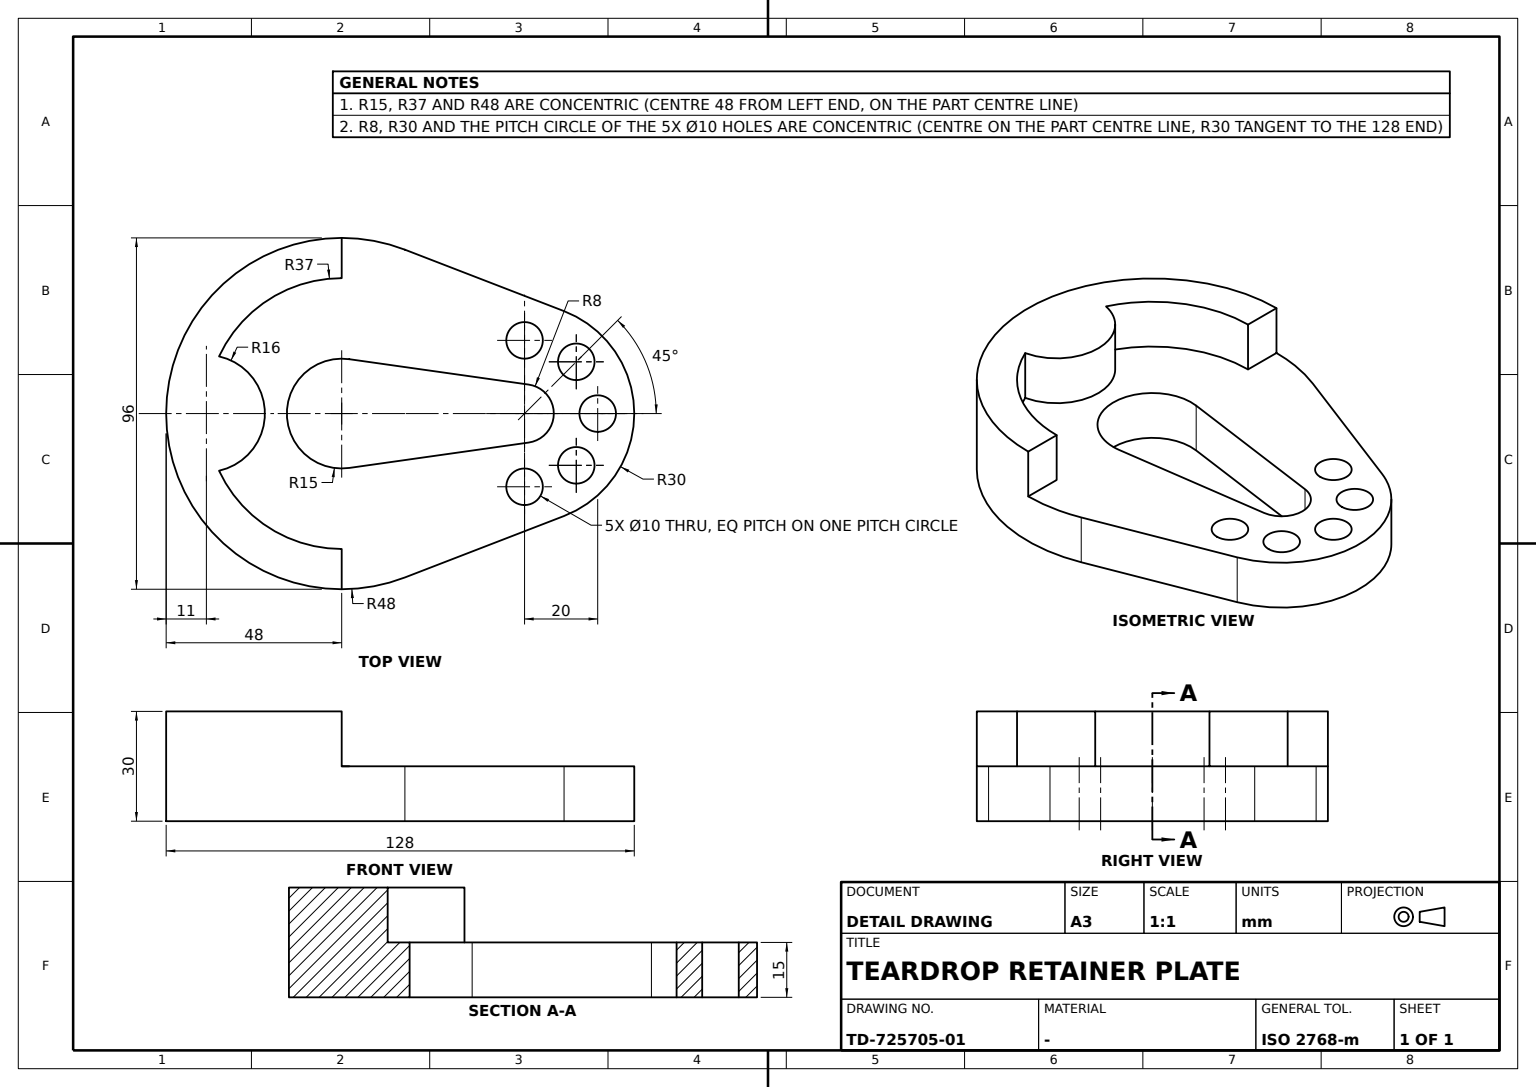
ISO-10303-21;
HEADER;
FILE_DESCRIPTION((''),'2;1');
FILE_NAME('','',(''),(''),'','','');
FILE_SCHEMA(('AUTOMOTIVE_DESIGN'));
ENDSEC;
DATA;
#1=APPLICATION_CONTEXT('');
#2=PRODUCT_CONTEXT('',#1,'mechanical');
#3=PRODUCT('','','',(#2));
#4=PRODUCT_DEFINITION_FORMATION('','',#3);
#5=PRODUCT_DEFINITION_CONTEXT('',#1,'design');
#6=PRODUCT_DEFINITION('','',#4,#5);
#7=PRODUCT_DEFINITION_SHAPE('','',#6);
#8=(LENGTH_UNIT()NAMED_UNIT(*)SI_UNIT(.MILLI.,.METRE.));
#9=(NAMED_UNIT(*)PLANE_ANGLE_UNIT()SI_UNIT($,.RADIAN.));
#10=(NAMED_UNIT(*)SI_UNIT($,.STERADIAN.)SOLID_ANGLE_UNIT());
#11=UNCERTAINTY_MEASURE_WITH_UNIT(LENGTH_MEASURE(0.005),#8,'distance_accuracy_value','');
#12=(GEOMETRIC_REPRESENTATION_CONTEXT(3)GLOBAL_UNCERTAINTY_ASSIGNED_CONTEXT((#11))GLOBAL_UNIT_ASSIGNED_CONTEXT((#8,#9,#10))REPRESENTATION_CONTEXT('',''));
#13=CARTESIAN_POINT('',(7.921212,51.12,0.));
#14=VERTEX_POINT('',#13);
#15=CARTESIAN_POINT('',(-7.921212,51.12,0.));
#16=VERTEX_POINT('',#15);
#17=CARTESIAN_POINT('',(0.,50.,0.));
#18=DIRECTION('',(0.,0.,1.));
#19=DIRECTION('',(1.,0.,0.));
#20=AXIS2_PLACEMENT_3D('',#17,#18,#19);
#21=CIRCLE('',#20,8.);
#22=EDGE_CURVE('',#14,#16,#21,.T.);
#23=ORIENTED_EDGE('',*,*,#22,.T.);
#24=CARTESIAN_POINT('',(-7.921212,51.12,-15.));
#25=VERTEX_POINT('',#24);
#26=CARTESIAN_POINT('',(-7.921212,51.12,-7.5));
#27=VECTOR('',#18,1000.);
#28=LINE('',#26,#27);
#29=EDGE_CURVE('',#16,#25,#28,.F.);
#30=ORIENTED_EDGE('',*,*,#29,.T.);
#31=CARTESIAN_POINT('',(7.921212,51.12,-15.));
#32=VERTEX_POINT('',#31);
#33=CARTESIAN_POINT('',(0.,50.,-15.));
#34=AXIS2_PLACEMENT_3D('',#33,#18,#19);
#35=CIRCLE('',#34,8.);
#36=EDGE_CURVE('',#32,#25,#35,.T.);
#37=ORIENTED_EDGE('',*,*,#36,.F.);
#38=CARTESIAN_POINT('',(7.921212,51.12,-7.5));
#39=LINE('',#38,#27);
#40=EDGE_CURVE('',#14,#32,#39,.F.);
#41=ORIENTED_EDGE('',*,*,#40,.F.);
#42=EDGE_LOOP('',(#23,#30,#37,#41));
#43=FACE_BOUND('',#42,.T.);
#44=CARTESIAN_POINT('',(0.,50.,-7.5));
#45=AXIS2_PLACEMENT_3D('',#44,#18,#19);
#46=CYLINDRICAL_SURFACE('',#45,8.);
#47=ADVANCED_FACE('',(#43),#46,.F.);
#48=CARTESIAN_POINT('',(19.142136,64.142136,-15.));
#49=VERTEX_POINT('',#48);
#50=CARTESIAN_POINT('',(14.142136,64.142136,-15.));
#51=AXIS2_PLACEMENT_3D('',#50,#18,#19);
#52=CIRCLE('',#51,5.);
#53=EDGE_CURVE('',#49,#49,#52,.T.);
#54=ORIENTED_EDGE('',*,*,#53,.T.);
#55=EDGE_LOOP('',(#54));
#56=FACE_BOUND('',#55,.T.);
#57=CARTESIAN_POINT('',(-44.781711,17.28,-15.));
#58=VERTEX_POINT('',#57);
#59=CARTESIAN_POINT('',(44.781711,17.28,-15.));
#60=VERTEX_POINT('',#59);
#61=CARTESIAN_POINT('',(0.,0.,-15.));
#62=AXIS2_PLACEMENT_3D('',#61,#18,#19);
#63=CIRCLE('',#62,48.);
#64=EDGE_CURVE('',#58,#60,#63,.T.);
#65=ORIENTED_EDGE('',*,*,#64,.F.);
#66=CARTESIAN_POINT('',(-27.988569,60.8,-15.));
#67=VERTEX_POINT('',#66);
#68=DIRECTION('',(0.36,0.932952303,0.));
#69=VECTOR('',#68,1000.);
#70=LINE('',#57,#69);
#71=EDGE_CURVE('',#58,#67,#70,.T.);
#72=ORIENTED_EDGE('',*,*,#71,.T.);
#73=CARTESIAN_POINT('',(27.988569,60.8,-15.));
#74=VERTEX_POINT('',#73);
#75=CIRCLE('',#34,30.);
#76=EDGE_CURVE('',#74,#67,#75,.T.);
#77=ORIENTED_EDGE('',*,*,#76,.F.);
#78=DIRECTION('',(0.36,-0.932952303,0.));
#79=VECTOR('',#78,1000.);
#80=LINE('',#73,#79);
#81=EDGE_CURVE('',#74,#60,#80,.T.);
#82=ORIENTED_EDGE('',*,*,#81,.T.);
#83=EDGE_LOOP('',(#65,#72,#77,#82));
#84=FACE_BOUND('',#83,.T.);
#85=CARTESIAN_POINT('',(-15.,50.,-15.));
#86=VERTEX_POINT('',#85);
#87=CARTESIAN_POINT('',(-20.,50.,-15.));
#88=AXIS2_PLACEMENT_3D('',#87,#18,#19);
#89=CIRCLE('',#88,5.);
#90=EDGE_CURVE('',#86,#86,#89,.T.);
#91=ORIENTED_EDGE('',*,*,#90,.T.);
#92=EDGE_LOOP('',(#91));
#93=FACE_BOUND('',#92,.T.);
#94=CARTESIAN_POINT('',(5.,70.,-15.));
#95=VERTEX_POINT('',#94);
#96=CARTESIAN_POINT('',(0.,70.,-15.));
#97=AXIS2_PLACEMENT_3D('',#96,#18,#19);
#98=CIRCLE('',#97,5.);
#99=EDGE_CURVE('',#95,#95,#98,.T.);
#100=ORIENTED_EDGE('',*,*,#99,.T.);
#101=EDGE_LOOP('',(#100));
#102=FACE_BOUND('',#101,.T.);
#103=CARTESIAN_POINT('',(25.,50.,-15.));
#104=VERTEX_POINT('',#103);
#105=CARTESIAN_POINT('',(20.,50.,-15.));
#106=AXIS2_PLACEMENT_3D('',#105,#18,#19);
#107=CIRCLE('',#106,5.);
#108=EDGE_CURVE('',#104,#104,#107,.T.);
#109=ORIENTED_EDGE('',*,*,#108,.T.);
#110=EDGE_LOOP('',(#109));
#111=FACE_BOUND('',#110,.T.);
#112=CARTESIAN_POINT('',(-9.142136,64.142136,-15.));
#113=VERTEX_POINT('',#112);
#114=CARTESIAN_POINT('',(-14.142136,64.142136,-15.));
#115=AXIS2_PLACEMENT_3D('',#114,#18,#19);
#116=CIRCLE('',#115,5.);
#117=EDGE_CURVE('',#113,#113,#116,.T.);
#118=ORIENTED_EDGE('',*,*,#117,.T.);
#119=EDGE_LOOP('',(#118));
#120=FACE_BOUND('',#119,.T.);
#121=CARTESIAN_POINT('',(-14.852273,2.1,-15.));
#122=VERTEX_POINT('',#121);
#123=CARTESIAN_POINT('',(14.852273,2.1,-15.));
#124=VERTEX_POINT('',#123);
#125=CIRCLE('',#62,15.);
#126=EDGE_CURVE('',#122,#124,#125,.T.);
#127=ORIENTED_EDGE('',*,*,#126,.T.);
#128=DIRECTION('',(0.14,-0.990151504,0.));
#129=VECTOR('',#128,1000.);
#130=LINE('',#31,#129);
#131=EDGE_CURVE('',#32,#124,#130,.T.);
#132=ORIENTED_EDGE('',*,*,#131,.F.);
#133=ORIENTED_EDGE('',*,*,#36,.T.);
#134=DIRECTION('',(0.14,0.990151504,0.));
#135=VECTOR('',#134,1000.);
#136=LINE('',#121,#135);
#137=EDGE_CURVE('',#122,#25,#136,.T.);
#138=ORIENTED_EDGE('',*,*,#137,.F.);
#139=EDGE_LOOP('',(#127,#132,#133,#138));
#140=FACE_BOUND('',#139,.T.);
#141=PLANE('',#62);
#142=ADVANCED_FACE('',(#56,#84,#93,#102,#111,#120,#140),#141,.F.);
#143=CARTESIAN_POINT('',(25.,50.,0.));
#144=VERTEX_POINT('',#143);
#145=CARTESIAN_POINT('',(20.,50.,0.));
#146=AXIS2_PLACEMENT_3D('',#145,#18,#19);
#147=CIRCLE('',#146,5.);
#148=EDGE_CURVE('',#144,#144,#147,.T.);
#149=ORIENTED_EDGE('',*,*,#148,.T.);
#150=EDGE_LOOP('',(#149));
#151=FACE_BOUND('',#150,.T.);
#152=ORIENTED_EDGE('',*,*,#108,.F.);
#153=EDGE_LOOP('',(#152));
#154=FACE_BOUND('',#153,.T.);
#155=CARTESIAN_POINT('',(20.,50.,-7.5));
#156=AXIS2_PLACEMENT_3D('',#155,#18,#19);
#157=CYLINDRICAL_SURFACE('',#156,5.);
#158=ADVANCED_FACE('',(#151,#154),#157,.F.);
#159=CARTESIAN_POINT('',(27.988569,60.8,0.));
#160=VERTEX_POINT('',#159);
#161=CARTESIAN_POINT('',(44.781711,17.28,0.));
#162=VERTEX_POINT('',#161);
#163=LINE('',#159,#79);
#164=EDGE_CURVE('',#160,#162,#163,.T.);
#165=ORIENTED_EDGE('',*,*,#164,.T.);
#166=CARTESIAN_POINT('',(44.781711,17.28,-7.5));
#167=LINE('',#166,#27);
#168=EDGE_CURVE('',#162,#60,#167,.F.);
#169=ORIENTED_EDGE('',*,*,#168,.T.);
#170=ORIENTED_EDGE('',*,*,#81,.F.);
#171=CARTESIAN_POINT('',(27.988569,60.8,-7.5));
#172=LINE('',#171,#27);
#173=EDGE_CURVE('',#160,#74,#172,.F.);
#174=ORIENTED_EDGE('',*,*,#173,.F.);
#175=EDGE_LOOP('',(#165,#169,#170,#174));
#176=FACE_BOUND('',#175,.T.);
#177=DIRECTION('',(0.932952303,0.36,0.));
#178=AXIS2_PLACEMENT_3D('',#159,#177,#78);
#179=PLANE('',#178);
#180=ADVANCED_FACE('',(#176),#179,.T.);
#181=ORIENTED_EDGE('',*,*,#71,.F.);
#182=CARTESIAN_POINT('',(-44.781711,17.28,0.));
#183=VERTEX_POINT('',#182);
#184=CARTESIAN_POINT('',(-44.781711,17.28,-7.5));
#185=LINE('',#184,#27);
#186=EDGE_CURVE('',#183,#58,#185,.F.);
#187=ORIENTED_EDGE('',*,*,#186,.F.);
#188=CARTESIAN_POINT('',(-27.988569,60.8,0.));
#189=VERTEX_POINT('',#188);
#190=LINE('',#182,#69);
#191=EDGE_CURVE('',#183,#189,#190,.T.);
#192=ORIENTED_EDGE('',*,*,#191,.T.);
#193=CARTESIAN_POINT('',(-27.988569,60.8,-7.5));
#194=LINE('',#193,#27);
#195=EDGE_CURVE('',#189,#67,#194,.F.);
#196=ORIENTED_EDGE('',*,*,#195,.T.);
#197=EDGE_LOOP('',(#181,#187,#192,#196));
#198=FACE_BOUND('',#197,.T.);
#199=DIRECTION('',(-0.932952303,0.36,0.));
#200=AXIS2_PLACEMENT_3D('',#182,#199,#68);
#201=PLANE('',#200);
#202=ADVANCED_FACE('',(#198),#201,.T.);
#203=CARTESIAN_POINT('',(15.621528,-33.540541,15.));
#204=VERTEX_POINT('',#203);
#205=CARTESIAN_POINT('',(-15.621528,-33.540541,15.));
#206=VERTEX_POINT('',#205);
#207=CARTESIAN_POINT('',(0.,-37.,15.));
#208=AXIS2_PLACEMENT_3D('',#207,#18,#19);
#209=CIRCLE('',#208,16.);
#210=EDGE_CURVE('',#204,#206,#209,.T.);
#211=ORIENTED_EDGE('',*,*,#210,.F.);
#212=CARTESIAN_POINT('',(15.621528,-33.540541,0.));
#213=VERTEX_POINT('',#212);
#214=LINE('',#212,#27);
#215=EDGE_CURVE('',#213,#204,#214,.T.);
#216=ORIENTED_EDGE('',*,*,#215,.F.);
#217=CARTESIAN_POINT('',(-15.621528,-33.540541,0.));
#218=VERTEX_POINT('',#217);
#219=CARTESIAN_POINT('',(0.,-37.,0.));
#220=AXIS2_PLACEMENT_3D('',#219,#18,#19);
#221=CIRCLE('',#220,16.);
#222=EDGE_CURVE('',#213,#218,#221,.T.);
#223=ORIENTED_EDGE('',*,*,#222,.T.);
#224=LINE('',#217,#27);
#225=EDGE_CURVE('',#218,#206,#224,.T.);
#226=ORIENTED_EDGE('',*,*,#225,.T.);
#227=EDGE_LOOP('',(#211,#216,#223,#226));
#228=FACE_BOUND('',#227,.T.);
#229=CARTESIAN_POINT('',(0.,-37.,7.5));
#230=AXIS2_PLACEMENT_3D('',#229,#18,#19);
#231=CYLINDRICAL_SURFACE('',#230,16.);
#232=ADVANCED_FACE('',(#228),#231,.T.);
#233=CARTESIAN_POINT('',(48.,0.,0.));
#234=VERTEX_POINT('',#233);
#235=CARTESIAN_POINT('',(48.,0.,15.));
#236=VERTEX_POINT('',#235);
#237=LINE('',#233,#27);
#238=EDGE_CURVE('',#234,#236,#237,.T.);
#239=ORIENTED_EDGE('',*,*,#238,.F.);
#240=CARTESIAN_POINT('',(37.,0.,0.));
#241=VERTEX_POINT('',#240);
#242=CARTESIAN_POINT('',(0.,0.,0.));
#243=DIRECTION('',(-1.,0.,0.));
#244=VECTOR('',#243,1000.);
#245=LINE('',#242,#244);
#246=EDGE_CURVE('',#234,#241,#245,.T.);
#247=ORIENTED_EDGE('',*,*,#246,.T.);
#248=CARTESIAN_POINT('',(37.,0.,15.));
#249=VERTEX_POINT('',#248);
#250=LINE('',#240,#27);
#251=EDGE_CURVE('',#241,#249,#250,.T.);
#252=ORIENTED_EDGE('',*,*,#251,.T.);
#253=CARTESIAN_POINT('',(0.,0.,15.));
#254=LINE('',#253,#244);
#255=EDGE_CURVE('',#236,#249,#254,.T.);
#256=ORIENTED_EDGE('',*,*,#255,.F.);
#257=EDGE_LOOP('',(#239,#247,#252,#256));
#258=FACE_BOUND('',#257,.T.);
#259=DIRECTION('',(0.,1.,0.));
#260=AXIS2_PLACEMENT_3D('',#233,#259,#243);
#261=PLANE('',#260);
#262=ADVANCED_FACE('',(#258),#261,.T.);
#263=CARTESIAN_POINT('',(-15.,50.,0.));
#264=VERTEX_POINT('',#263);
#265=CARTESIAN_POINT('',(-20.,50.,0.));
#266=AXIS2_PLACEMENT_3D('',#265,#18,#19);
#267=CIRCLE('',#266,5.);
#268=EDGE_CURVE('',#264,#264,#267,.T.);
#269=ORIENTED_EDGE('',*,*,#268,.T.);
#270=EDGE_LOOP('',(#269));
#271=FACE_BOUND('',#270,.T.);
#272=ORIENTED_EDGE('',*,*,#90,.F.);
#273=EDGE_LOOP('',(#272));
#274=FACE_BOUND('',#273,.T.);
#275=CARTESIAN_POINT('',(-20.,50.,-7.5));
#276=AXIS2_PLACEMENT_3D('',#275,#18,#19);
#277=CYLINDRICAL_SURFACE('',#276,5.);
#278=ADVANCED_FACE('',(#271,#274),#277,.F.);
#279=ORIENTED_EDGE('',*,*,#29,.F.);
#280=CARTESIAN_POINT('',(-14.852273,2.1,0.));
#281=VERTEX_POINT('',#280);
#282=LINE('',#280,#135);
#283=EDGE_CURVE('',#281,#16,#282,.T.);
#284=ORIENTED_EDGE('',*,*,#283,.F.);
#285=CARTESIAN_POINT('',(-14.852273,2.1,-7.5));
#286=LINE('',#285,#27);
#287=EDGE_CURVE('',#281,#122,#286,.F.);
#288=ORIENTED_EDGE('',*,*,#287,.T.);
#289=ORIENTED_EDGE('',*,*,#137,.T.);
#290=EDGE_LOOP('',(#279,#284,#288,#289));
#291=FACE_BOUND('',#290,.T.);
#292=DIRECTION('',(-0.990151504,0.14,0.));
#293=AXIS2_PLACEMENT_3D('',#280,#292,#134);
#294=PLANE('',#293);
#295=ADVANCED_FACE('',(#291),#294,.F.);
#296=ORIENTED_EDGE('',*,*,#131,.T.);
#297=CARTESIAN_POINT('',(14.852273,2.1,0.));
#298=VERTEX_POINT('',#297);
#299=CARTESIAN_POINT('',(14.852273,2.1,-7.5));
#300=LINE('',#299,#27);
#301=EDGE_CURVE('',#298,#124,#300,.F.);
#302=ORIENTED_EDGE('',*,*,#301,.F.);
#303=LINE('',#13,#129);
#304=EDGE_CURVE('',#14,#298,#303,.T.);
#305=ORIENTED_EDGE('',*,*,#304,.F.);
#306=ORIENTED_EDGE('',*,*,#40,.T.);
#307=EDGE_LOOP('',(#296,#302,#305,#306));
#308=FACE_BOUND('',#307,.T.);
#309=DIRECTION('',(0.990151504,0.14,0.));
#310=AXIS2_PLACEMENT_3D('',#13,#309,#128);
#311=PLANE('',#310);
#312=ADVANCED_FACE('',(#308),#311,.F.);
#313=ORIENTED_EDGE('',*,*,#99,.F.);
#314=EDGE_LOOP('',(#313));
#315=FACE_BOUND('',#314,.T.);
#316=CARTESIAN_POINT('',(5.,70.,0.));
#317=VERTEX_POINT('',#316);
#318=CARTESIAN_POINT('',(0.,70.,0.));
#319=AXIS2_PLACEMENT_3D('',#318,#18,#19);
#320=CIRCLE('',#319,5.);
#321=EDGE_CURVE('',#317,#317,#320,.T.);
#322=ORIENTED_EDGE('',*,*,#321,.T.);
#323=EDGE_LOOP('',(#322));
#324=FACE_BOUND('',#323,.T.);
#325=CARTESIAN_POINT('',(0.,70.,-7.5));
#326=AXIS2_PLACEMENT_3D('',#325,#18,#19);
#327=CYLINDRICAL_SURFACE('',#326,5.);
#328=ADVANCED_FACE('',(#315,#324),#327,.F.);
#329=CARTESIAN_POINT('',(-37.,0.,0.));
#330=VERTEX_POINT('',#329);
#331=CARTESIAN_POINT('',(-48.,0.,0.));
#332=VERTEX_POINT('',#331);
#333=EDGE_CURVE('',#330,#332,#245,.T.);
#334=ORIENTED_EDGE('',*,*,#333,.T.);
#335=CARTESIAN_POINT('',(-48.,0.,15.));
#336=VERTEX_POINT('',#335);
#337=LINE('',#331,#27);
#338=EDGE_CURVE('',#332,#336,#337,.T.);
#339=ORIENTED_EDGE('',*,*,#338,.T.);
#340=CARTESIAN_POINT('',(-37.,0.,15.));
#341=VERTEX_POINT('',#340);
#342=EDGE_CURVE('',#341,#336,#254,.T.);
#343=ORIENTED_EDGE('',*,*,#342,.F.);
#344=LINE('',#329,#27);
#345=EDGE_CURVE('',#330,#341,#344,.T.);
#346=ORIENTED_EDGE('',*,*,#345,.F.);
#347=EDGE_LOOP('',(#334,#339,#343,#346));
#348=FACE_BOUND('',#347,.T.);
#349=ADVANCED_FACE('',(#348),#261,.T.);
#350=AXIS2_PLACEMENT_3D('',#242,#18,#19);
#351=CIRCLE('',#350,15.);
#352=EDGE_CURVE('',#281,#298,#351,.T.);
#353=ORIENTED_EDGE('',*,*,#352,.T.);
#354=ORIENTED_EDGE('',*,*,#301,.T.);
#355=ORIENTED_EDGE('',*,*,#126,.F.);
#356=ORIENTED_EDGE('',*,*,#287,.F.);
#357=EDGE_LOOP('',(#353,#354,#355,#356));
#358=FACE_BOUND('',#357,.T.);
#359=CARTESIAN_POINT('',(0.,0.,-7.5));
#360=AXIS2_PLACEMENT_3D('',#359,#18,#19);
#361=CYLINDRICAL_SURFACE('',#360,15.);
#362=ADVANCED_FACE('',(#358),#361,.F.);
#363=ORIENTED_EDGE('',*,*,#246,.F.);
#364=CIRCLE('',#350,48.);
#365=EDGE_CURVE('',#234,#162,#364,.T.);
#366=ORIENTED_EDGE('',*,*,#365,.T.);
#367=ORIENTED_EDGE('',*,*,#164,.F.);
#368=CIRCLE('',#20,30.);
#369=EDGE_CURVE('',#160,#189,#368,.T.);
#370=ORIENTED_EDGE('',*,*,#369,.T.);
#371=ORIENTED_EDGE('',*,*,#191,.F.);
#372=EDGE_CURVE('',#183,#332,#364,.T.);
#373=ORIENTED_EDGE('',*,*,#372,.T.);
#374=ORIENTED_EDGE('',*,*,#333,.F.);
#375=CIRCLE('',#350,37.);
#376=EDGE_CURVE('',#330,#218,#375,.T.);
#377=ORIENTED_EDGE('',*,*,#376,.T.);
#378=ORIENTED_EDGE('',*,*,#222,.F.);
#379=EDGE_CURVE('',#213,#241,#375,.T.);
#380=ORIENTED_EDGE('',*,*,#379,.T.);
#381=EDGE_LOOP('',(#363,#366,#367,#370,#371,#373,#374,#377,#378,#380));
#382=FACE_BOUND('',#381,.T.);
#383=ORIENTED_EDGE('',*,*,#283,.T.);
#384=ORIENTED_EDGE('',*,*,#22,.F.);
#385=ORIENTED_EDGE('',*,*,#304,.T.);
#386=ORIENTED_EDGE('',*,*,#352,.F.);
#387=EDGE_LOOP('',(#383,#384,#385,#386));
#388=FACE_BOUND('',#387,.T.);
#389=CARTESIAN_POINT('',(-9.142136,64.142136,0.));
#390=VERTEX_POINT('',#389);
#391=CARTESIAN_POINT('',(-14.142136,64.142136,0.));
#392=AXIS2_PLACEMENT_3D('',#391,#18,#19);
#393=CIRCLE('',#392,5.);
#394=EDGE_CURVE('',#390,#390,#393,.T.);
#395=ORIENTED_EDGE('',*,*,#394,.F.);
#396=EDGE_LOOP('',(#395));
#397=FACE_BOUND('',#396,.T.);
#398=ORIENTED_EDGE('',*,*,#148,.F.);
#399=EDGE_LOOP('',(#398));
#400=FACE_BOUND('',#399,.T.);
#401=ORIENTED_EDGE('',*,*,#268,.F.);
#402=EDGE_LOOP('',(#401));
#403=FACE_BOUND('',#402,.T.);
#404=CARTESIAN_POINT('',(19.142136,64.142136,0.));
#405=VERTEX_POINT('',#404);
#406=CARTESIAN_POINT('',(14.142136,64.142136,0.));
#407=AXIS2_PLACEMENT_3D('',#406,#18,#19);
#408=CIRCLE('',#407,5.);
#409=EDGE_CURVE('',#405,#405,#408,.T.);
#410=ORIENTED_EDGE('',*,*,#409,.F.);
#411=EDGE_LOOP('',(#410));
#412=FACE_BOUND('',#411,.T.);
#413=ORIENTED_EDGE('',*,*,#321,.F.);
#414=EDGE_LOOP('',(#413));
#415=FACE_BOUND('',#414,.T.);
#416=PLANE('',#350);
#417=ADVANCED_FACE('',(#382,#388,#397,#400,#403,#412,#415),#416,.T.);
#418=ORIENTED_EDGE('',*,*,#409,.T.);
#419=EDGE_LOOP('',(#418));
#420=FACE_BOUND('',#419,.T.);
#421=ORIENTED_EDGE('',*,*,#53,.F.);
#422=EDGE_LOOP('',(#421));
#423=FACE_BOUND('',#422,.T.);
#424=CARTESIAN_POINT('',(14.142136,64.142136,-7.5));
#425=AXIS2_PLACEMENT_3D('',#424,#18,#19);
#426=CYLINDRICAL_SURFACE('',#425,5.);
#427=ADVANCED_FACE('',(#420,#423),#426,.F.);
#428=ORIENTED_EDGE('',*,*,#251,.F.);
#429=ORIENTED_EDGE('',*,*,#379,.F.);
#430=ORIENTED_EDGE('',*,*,#215,.T.);
#431=AXIS2_PLACEMENT_3D('',#253,#18,#19);
#432=CIRCLE('',#431,37.);
#433=EDGE_CURVE('',#204,#249,#432,.T.);
#434=ORIENTED_EDGE('',*,*,#433,.T.);
#435=EDGE_LOOP('',(#428,#429,#430,#434));
#436=FACE_BOUND('',#435,.T.);
#437=CARTESIAN_POINT('',(0.,0.,7.5));
#438=AXIS2_PLACEMENT_3D('',#437,#18,#19);
#439=CYLINDRICAL_SURFACE('',#438,37.);
#440=ADVANCED_FACE('',(#436),#439,.F.);
#441=ORIENTED_EDGE('',*,*,#117,.F.);
#442=EDGE_LOOP('',(#441));
#443=FACE_BOUND('',#442,.T.);
#444=ORIENTED_EDGE('',*,*,#394,.T.);
#445=EDGE_LOOP('',(#444));
#446=FACE_BOUND('',#445,.T.);
#447=CARTESIAN_POINT('',(-14.142136,64.142136,-7.5));
#448=AXIS2_PLACEMENT_3D('',#447,#18,#19);
#449=CYLINDRICAL_SURFACE('',#448,5.);
#450=ADVANCED_FACE('',(#443,#446),#449,.F.);
#451=ORIENTED_EDGE('',*,*,#238,.T.);
#452=CIRCLE('',#431,48.);
#453=EDGE_CURVE('',#336,#236,#452,.T.);
#454=ORIENTED_EDGE('',*,*,#453,.F.);
#455=ORIENTED_EDGE('',*,*,#338,.F.);
#456=ORIENTED_EDGE('',*,*,#372,.F.);
#457=ORIENTED_EDGE('',*,*,#186,.T.);
#458=ORIENTED_EDGE('',*,*,#64,.T.);
#459=ORIENTED_EDGE('',*,*,#168,.F.);
#460=ORIENTED_EDGE('',*,*,#365,.F.);
#461=EDGE_LOOP('',(#451,#454,#455,#456,#457,#458,#459,#460));
#462=FACE_BOUND('',#461,.T.);
#463=CYLINDRICAL_SURFACE('',#360,48.);
#464=ADVANCED_FACE('',(#462),#463,.T.);
#465=ORIENTED_EDGE('',*,*,#195,.F.);
#466=ORIENTED_EDGE('',*,*,#369,.F.);
#467=ORIENTED_EDGE('',*,*,#173,.T.);
#468=ORIENTED_EDGE('',*,*,#76,.T.);
#469=EDGE_LOOP('',(#465,#466,#467,#468));
#470=FACE_BOUND('',#469,.T.);
#471=CYLINDRICAL_SURFACE('',#45,30.);
#472=ADVANCED_FACE('',(#470),#471,.T.);
#473=ORIENTED_EDGE('',*,*,#453,.T.);
#474=ORIENTED_EDGE('',*,*,#255,.T.);
#475=ORIENTED_EDGE('',*,*,#433,.F.);
#476=ORIENTED_EDGE('',*,*,#210,.T.);
#477=EDGE_CURVE('',#341,#206,#432,.T.);
#478=ORIENTED_EDGE('',*,*,#477,.F.);
#479=ORIENTED_EDGE('',*,*,#342,.T.);
#480=EDGE_LOOP('',(#473,#474,#475,#476,#478,#479));
#481=FACE_BOUND('',#480,.T.);
#482=PLANE('',#431);
#483=ADVANCED_FACE('',(#481),#482,.T.);
#484=ORIENTED_EDGE('',*,*,#477,.T.);
#485=ORIENTED_EDGE('',*,*,#225,.F.);
#486=ORIENTED_EDGE('',*,*,#376,.F.);
#487=ORIENTED_EDGE('',*,*,#345,.T.);
#488=EDGE_LOOP('',(#484,#485,#486,#487));
#489=FACE_BOUND('',#488,.T.);
#490=ADVANCED_FACE('',(#489),#439,.F.);
#491=CLOSED_SHELL('',(#47,#142,#158,#180,#202,#232,#262,#278,#295,#312,#328,#349,#362,#417,#427,#440,#450,#464,#472,#483,#490));
#492=MANIFOLD_SOLID_BREP('',#491);
#493=ADVANCED_BREP_SHAPE_REPRESENTATION('',(#492),#12);
#494=SHAPE_DEFINITION_REPRESENTATION(#7,#493);
ENDSEC;
END-ISO-10303-21;
